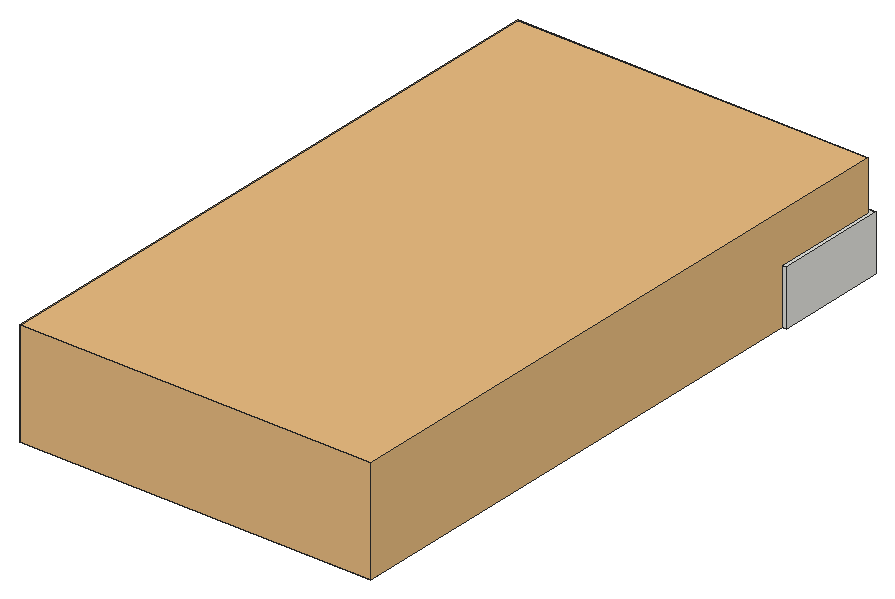
# SketchUp Ruby script. Lengths in inches.
U = 1.inch
M = Sketchup.active_model
def pt(a) = Geom::Point3d.new(a.map { |v| v * U })
def face(e, loops, mat)
  f = e.add_face(loops[0].map { |a| pt(a) })
  loops[1..].each { |l| e.add_face(l.map { |a| pt(a) }).erase! }
  f.material = f.back_material = mat if mat
  f
end
# faces: each face lists its corners as indices into pts; further lists are holes
def faces(e, pts, list, mat = nil) = list.each { |f| face(e, (f[0].is_a?(Array) ? f : [f]).map { |l| l.map { |i| pts[i] } }, mat) }
# xy, xz, yz: faces in a plane at the given z, y or x. An outline is a flat list of corners, or four numbers for a rectangle; further outlines are holes
def ring(l) = l.size == 4 ? [[l[0], l[1]], [l[2], l[1]], [l[2], l[3]], [l[0], l[3]]] : l.each_slice(2).to_a
def flat(e, list, mat, &to3) = list.each { |f| face(e, (f[0].is_a?(Array) ? f : [f]).map { |l| ring(l).map { |u, v| to3.(u, v) } }, mat) }
def xy(e, z, list, mat = nil) = flat(e, list, mat) { |x, y| [x, y, z] }
def xz(e, y, list, mat = nil) = flat(e, list, mat) { |x, z| [x, y, z] }
def yz(e, x, list, mat = nil) = flat(e, list, mat) { |y, z| [x, y, z] }
def lines(e, pts, list) = list.each { |a, b| e.add_line(pt(pts[a]), pt(pts[b])) }
# prism: a flat outline (further loops are holes) pulled along v
def prism(e, loops, v, mat = nil)
  f = face(e, loops, mat); d = Geom::Vector3d.new(v.map { |x| x * U })
  f.pushpull(f.normal.samedirection?(d) ? d.length : -d.length)
end
def box(e, o, s, mat = nil) = prism(e, [[o, [o[0] + s[0], o[1], o[2]], [o[0] + s[0], o[1] + s[1], o[2]], [o[0], o[1] + s[1], o[2]]]], [0, 0, s[2]], mat)
def at(x, y, z, deg = 0) = Geom::Transformation.translation(pt([x, y, z])) * Geom::Transformation.rotation(ORIGIN, Z_AXIS, deg.degrees)
def axes(o, x, y, z) = Geom::Transformation.new([*x, 0, *y, 0, *z, 0, *pt(o).to_a, 1])
def part(name) = M.definitions.add(name)
# library, detail: a bought-in or finely detailed component or shape, given as its bounding box
def library(name, o, s) = part(name).tap { |d| box(d.entities, o, s) }
def detail(e, o, s) = box(e.add_group.entities, o, s)
def put(e, d, t, mat = nil) = e.add_instance(d, t).tap { |i| i.material = mat if mat }
def group(e, t, mat = nil) = e.add_group.tap { |g| g.transformation = t; g.material = mat if mat }.entities
root = M.entities
c1 = library("Sitting room",[-531.73,-1115.13,0],[753.73,1337.13,224.98])
xy(root,0,[[[0,0,240,240],[9,9,231,231]]])
xy(root,120,[[[0,0,240,240],[9,9,231,231]]])
xz(root,0,[[0,0,240,120]])
xz(root,231,[[9,0,231,120]])
xz(root,240,[[0,0,240,120]])
yz(root,0,[[0,0,240,120]])
yz(root,9,[[9,0,231,120]])
yz(root,240,[[0,0,240,120]])
put(root,c1,at(9,9,0))
